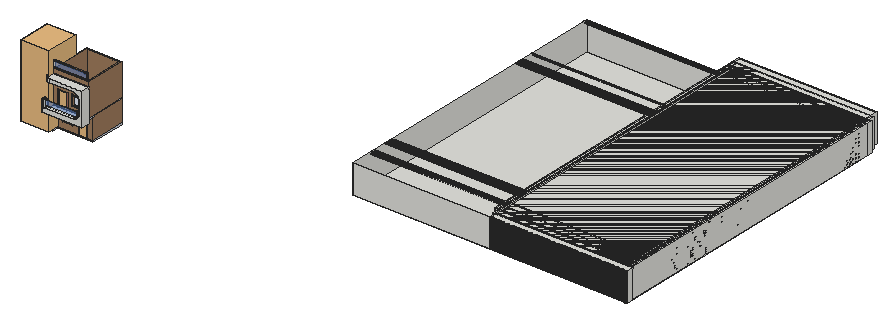
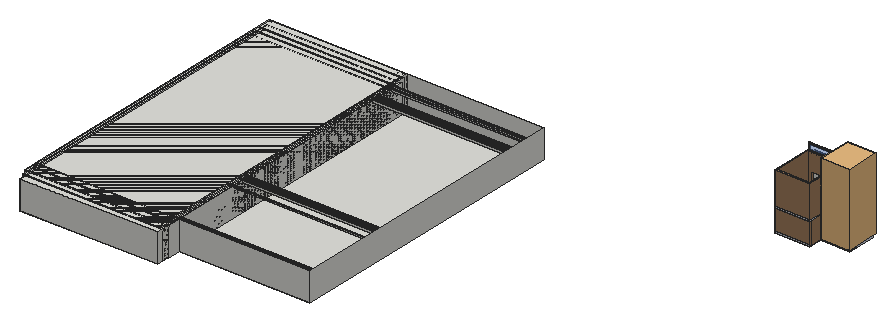
# SketchUp Ruby script. Lengths in inches.
U = 1.inch
M = Sketchup.active_model
def pt(a) = Geom::Point3d.new(a.map { |v| v * U })
def face(e, loops, mat)
  f = e.add_face(loops[0].map { |a| pt(a) })
  loops[1..].each { |l| e.add_face(l.map { |a| pt(a) }).erase! }
  f.material = f.back_material = mat if mat
  f
end
# faces: each face lists its corners as indices into pts; further lists are holes
def faces(e, pts, list, mat = nil) = list.each { |f| face(e, (f[0].is_a?(Array) ? f : [f]).map { |l| l.map { |i| pts[i] } }, mat) }
# xy, xz, yz: faces in a plane at the given z, y or x. An outline is a flat list of corners, or four numbers for a rectangle; further outlines are holes
def ring(l) = l.size == 4 ? [[l[0], l[1]], [l[2], l[1]], [l[2], l[3]], [l[0], l[3]]] : l.each_slice(2).to_a
def flat(e, list, mat, &to3) = list.each { |f| face(e, (f[0].is_a?(Array) ? f : [f]).map { |l| ring(l).map { |u, v| to3.(u, v) } }, mat) }
def xy(e, z, list, mat = nil) = flat(e, list, mat) { |x, y| [x, y, z] }
def xz(e, y, list, mat = nil) = flat(e, list, mat) { |x, z| [x, y, z] }
def yz(e, x, list, mat = nil) = flat(e, list, mat) { |y, z| [x, y, z] }
def lines(e, pts, list) = list.each { |a, b| e.add_line(pt(pts[a]), pt(pts[b])) }
# prism: a flat outline (further loops are holes) pulled along v
def prism(e, loops, v, mat = nil)
  f = face(e, loops, mat); d = Geom::Vector3d.new(v.map { |x| x * U })
  f.pushpull(f.normal.samedirection?(d) ? d.length : -d.length)
end
def box(e, o, s, mat = nil) = prism(e, [[o, [o[0] + s[0], o[1], o[2]], [o[0] + s[0], o[1] + s[1], o[2]], [o[0], o[1] + s[1], o[2]]]], [0, 0, s[2]], mat)
def at(x, y, z, deg = 0) = Geom::Transformation.translation(pt([x, y, z])) * Geom::Transformation.rotation(ORIGIN, Z_AXIS, deg.degrees)
def axes(o, x, y, z) = Geom::Transformation.new([*x, 0, *y, 0, *z, 0, *pt(o).to_a, 1])
def part(name) = M.definitions.add(name)
# library, detail: a bought-in or finely detailed component or shape, given as its bounding box
def library(name, o, s) = part(name).tap { |d| box(d.entities, o, s) }
def detail(e, o, s) = box(e.add_group.entities, o, s)
def put(e, d, t, mat = nil) = e.add_instance(d, t).tap { |i| i.material = mat if mat }
def group(e, t, mat = nil) = e.add_group.tap { |g| g.transformation = t; g.material = mat if mat }.entities
root = M.entities
M.materials.add("[Cladding Siding Tan]").color = [162, 126, 95]
M.materials.add("[Marble Carrara Floor Tile]").color = [204, 208, 219]
M.materials.add("[Stone Flagstone Ashlar]").color = [175, 116, 102]
M.materials.add("[Translucent Glass Blue]").color = [100, 149, 237]
M.materials["[Translucent Glass Blue]"].alpha = 0.5
c1 = part("Group478\#1")
prism(c1.entities,[[[385.16,-80.25,5.875],[385.16,-76.86,0],[385.16,-75.67,0],[385.16,-79.0625,5.875]]],[-770.3125,0,0])
c2 = part("Group479\#1")
prism(c2.entities,[[[385.16,-76.3125,5.875],[385.16,-72.92,0],[385.16,-71.73,0],[385.16,-75.125,5.875]]],[-770.3125,0,0])
c3 = part("Group480\#1")
prism(c3.entities,[[[385.16,-68.98,0],[385.16,-67.8,0],[385.16,-71.1875,5.875],[385.16,-72.375,5.875]]],[-770.3125,0,0])
c4 = part("Group481\#1")
prism(c4.entities,[[[-385.16,-63.86,0],[-385.16,-65.05,0],[-385.16,-68.4375,5.875],[-385.16,-67.25,5.875]]],[770.3125,0,0])
c5 = part("Group482\#1")
prism(c5.entities,[[[-385.16,-59.92,0],[-385.16,-61.11,0],[-385.16,-64.5,5.875],[-385.16,-63.3125,5.875]]],[770.3125,0,0])
c6 = part("Group483\#1")
prism(c6.entities,[[[385.16,-59.375,5.875],[385.16,-60.5625,5.875],[385.16,-57.17,0],[385.16,-55.98,0]]],[-770.3125,0,0])
c7 = part("Group484\#1")
prism(c7.entities,[[[385.16,-56.625,5.875],[385.16,-53.23,0],[385.16,-52.05,0],[385.16,-55.4375,5.875]]],[-770.3125,0,0])
c8 = part("Group485\#1")
prism(c8.entities,[[[385.16,-52.6875,5.875],[385.16,-49.3,0],[385.16,-48.11,0],[385.16,-51.5,5.875]]],[-770.3125,0,0])
c9 = part("Group486\#1")
prism(c9.entities,[[[-385.16,-48.75,5.875],[-385.16,-47.5625,5.875],[-385.16,-44.17,0],[-385.16,-45.36,0]]],[770.3125,0,0])
c10 = part("Group487\#1")
prism(c10.entities,[[[-385.16,-41.42,0],[-385.16,-44.8125,5.875],[-385.16,-43.625,5.875],[-385.16,-40.23,0]]],[770.3125,0,0])
c11 = part("Group488\#1")
prism(c11.entities,[[[385.16,-37.48,0],[385.16,-36.3,0],[385.16,-39.6875,5.875],[385.16,-40.875,5.875]]],[-770.3125,0,0])
c12 = part("Group489\#1")
prism(c12.entities,[[[385.16,-33.55,0],[385.16,-32.36,0],[385.16,-35.75,5.875],[385.16,-36.9375,5.875]]],[-770.3125,0,0])
c13 = part("Group490\#1")
prism(c13.entities,[[[385.16,-33,5.875],[385.16,-29.61,0],[385.16,-28.42,0],[385.16,-31.8125,5.875]]],[-770.3125,0,0])
c14 = part("Group491\#1")
prism(c14.entities,[[[385.16,-24.48,0],[385.16,-27.875,5.875],[385.16,-29.0625,5.875],[385.16,-25.67,0]]],[-770.3125,0,0])
c15 = part("Group492\#1")
prism(c15.entities,[[[-385.16,-25.125,5.875],[-385.16,-23.9375,5.875],[-385.16,-20.55,0],[-385.16,-21.73,0]]],[770.3125,0,0])
c16 = part("Group493\#1")
prism(c16.entities,[[[385.16,-21.1875,5.875],[385.16,-17.8,0],[385.16,-16.61,0],[385.16,-20,5.875]]],[-770.3125,0,0])
c17 = part("Group494\#1")
prism(c17.entities,[[[385.16,-13.86,0],[385.16,-12.67,0],[385.16,-16.0625,5.875],[385.16,-17.25,5.875]]],[-770.3125,0,0])
c18 = part("Group495\#1")
prism(c18.entities,[[[-385.16,-13.3125,5.875],[-385.16,-12.125,5.875],[-385.16,-8.73,0],[-385.16,-9.92,0]]],[770.3125,0,0])
c19 = part("Group496\#1")
prism(c19.entities,[[[385.16,-9.375,5.875],[385.16,-5.98,0],[385.16,-4.8,0],[385.16,-8.1875,5.875]]],[-770.3125,0,0])
c20 = part("Group497\#1")
prism(c20.entities,[[[385.16,-0.86,0],[385.16,-4.25,5.875],[385.16,-5.4375,5.875],[385.16,-2.05,0]]],[-770.3125,0,0])
c21 = part("Group498\#1")
prism(c21.entities,[[[-385.16,-1.5,5.875],[-385.16,-0.3125,5.875],[-385.16,3.08,0],[-385.16,1.89,0]]],[770.3125,0,0])
c22 = part("Group499\#1")
prism(c22.entities,[[[385.16,5.83,0],[385.16,7.02,0],[385.16,3.625,5.875],[385.16,2.4375,5.875]]],[-770.3125,0,0])
c23 = part("Group500\#1")
prism(c23.entities,[[[-385.16,9.77,0],[-385.16,6.375,5.875],[-385.16,7.5625,5.875],[-385.16,10.95,0]]],[770.3125,0,0])
c24 = part("Group501\#1")
prism(c24.entities,[[[-385.16,14.89,0],[-385.16,13.7,0],[-385.16,10.3125,5.875],[-385.16,11.5,5.875]]],[770.3125,0,0])
c25 = part("Group502\#1")
prism(c25.entities,[[[-385.16,15.4375,5.875],[-385.16,18.83,0],[-385.16,17.64,0],[-385.16,14.25,5.875]]],[770.3125,0,0])
c26 = part("Group503\#1")
prism(c26.entities,[[[385.16,19.375,5.875],[385.16,18.1875,5.875],[385.16,21.58,0],[385.16,22.77,0]]],[-770.3125,0,0])
c27 = part("Group504\#1")
prism(c27.entities,[[[-385.16,26.7,0],[-385.16,25.52,0],[-385.16,22.125,5.875],[-385.16,23.3125,5.875]]],[770.3125,0,0])
c28 = part("Group505\#1")
prism(c28.entities,[[[385.16,29.45,0],[385.16,30.64,0],[385.16,27.25,5.875],[385.16,26.0625,5.875]]],[-770.3125,0,0])
c29 = part("Group506\#1")
prism(c29.entities,[[[-385.16,33.39,0],[-385.16,30,5.875],[-385.16,31.1875,5.875],[-385.16,34.58,0]]],[770.3125,0,0])
c30 = part("Group507\#1")
prism(c30.entities,[[[385.16,33.9375,5.875],[385.16,37.33,0],[385.16,38.52,0],[385.16,35.125,5.875]]],[-770.3125,0,0])
c31 = part("Group508\#1")
prism(c31.entities,[[[-385.16,42.45,0],[-385.16,41.27,0],[-385.16,37.875,5.875],[-385.16,39.0625,5.875]]],[770.3125,0,0])
c32 = part("Group509\#1")
prism(c32.entities,[[[385.16,46.39,0],[385.16,43,5.875],[385.16,41.8125,5.875],[385.16,45.2,0]]],[-770.3125,0,0])
c33 = part("Group510\#1")
prism(c33.entities,[[[-385.16,49.14,0],[-385.16,45.75,5.875],[-385.16,46.9375,5.875],[-385.16,50.33,0]]],[770.3125,0,0])
c34 = part("Group511\#1")
prism(c34.entities,[[[385.16,50.875,5.875],[385.16,49.6875,5.875],[385.16,53.08,0],[385.16,54.27,0]]],[-770.3125,0,0])
c35 = part("Group512\#1")
prism(c35.entities,[[[385.16,54.8125,5.875],[385.16,53.625,5.875],[385.16,57.02,0],[385.16,58.2,0]]],[-770.3125,0,0])
c36 = part("Group513\#1")
prism(c36.entities,[[[385.16,62.14,0],[385.16,58.75,5.875],[385.16,57.5625,5.875],[385.16,60.95,0]]],[-770.3125,0,0])
c37 = part("Group514\#1")
prism(c37.entities,[[[-385.16,62.6875,5.875],[-385.16,66.08,0],[-385.16,64.89,0],[-385.16,61.5,5.875]]],[770.3125,0,0])
c38 = part("Group515\#1")
prism(c38.entities,[[[-385.16,70.02,0],[-385.16,68.83,0],[-385.16,65.4375,5.875],[-385.16,66.625,5.875]]],[770.3125,0,0])
c39 = part("Group516\#1")
prism(c39.entities,[[[385.16,72.77,0],[385.16,73.95,0],[385.16,70.5625,5.875],[385.16,69.375,5.875]]],[-770.3125,0,0])
c40 = part("Group517\#1")
prism(c40.entities,[[[385.16,76.7,0],[385.16,77.89,0],[385.16,74.5,5.875],[385.16,73.3125,5.875]]],[-770.3125,0,0])
c41 = part("Group518\#1")
xy(c41.entities,5.875,[[-385.16,77.25,385.16,78.4375]])
p = [[385.16,77.25,5.875],[-385.16,77.25,5.875],[-385.16,80.25,0.68],[385.16,80.25,0.68],[-385.16,78.4375,5.875],[385.16,78.4375,5.875],
  [385.16,80.25,2.74],[-385.16,80.25,2.74]]
faces(c41.entities,p,[[0,1,2,3],[4,5,6,7]])
c42 = part("Group476\#2")
put(c42.entities,c1,at(0,0,0))
put(c42.entities,c2,at(0,0,0))
put(c42.entities,c3,at(0,0,0))
put(c42.entities,c4,at(0,0,0))
put(c42.entities,c5,at(0,0,0))
put(c42.entities,c6,at(0,0,0))
put(c42.entities,c7,at(0,0,0))
put(c42.entities,c8,at(0,0,0))
put(c42.entities,c9,at(0,0,0))
put(c42.entities,c10,at(0,0,0))
put(c42.entities,c11,at(0,0,0))
put(c42.entities,c12,at(0,0,0))
put(c42.entities,c13,at(0,0,0))
put(c42.entities,c14,at(0,0,0))
put(c42.entities,c15,at(0,0,0))
put(c42.entities,c16,at(0,0,0))
put(c42.entities,c17,at(0,0,0))
put(c42.entities,c18,at(0,0,0))
put(c42.entities,c19,at(0,0,0))
put(c42.entities,c20,at(0,0,0))
put(c42.entities,c21,at(0,0,0))
put(c42.entities,c22,at(0,0,0))
put(c42.entities,c23,at(0,0,0))
put(c42.entities,c24,at(0,0,0))
put(c42.entities,c25,at(0,0,0))
put(c42.entities,c26,at(0,0,0))
put(c42.entities,c27,at(0,0,0))
put(c42.entities,c28,at(0,0,0))
put(c42.entities,c29,at(0,0,0))
put(c42.entities,c30,at(0,0,0))
put(c42.entities,c31,at(0,0,0))
put(c42.entities,c32,at(0,0,0))
put(c42.entities,c33,at(0,0,0))
put(c42.entities,c34,at(0,0,0))
put(c42.entities,c35,at(0,0,0))
put(c42.entities,c36,at(0,0,0))
put(c42.entities,c37,at(0,0,0))
put(c42.entities,c38,at(0,0,0))
put(c42.entities,c39,at(0,0,0))
put(c42.entities,c40,at(0,0,0))
put(c42.entities,c41,at(0,0,0))
c43 = library("Group1\#1",[84,59.0625,0],[162,188.875,405.6875])
c44 = library("Group\#3",[0,0,0],[54.125,9.07,48])
c45 = library("Group\#4",[0,0,0],[48.61,10.47,82])
c46 = part("Group14\#2")
xy(c46.entities,120,[[246,116.375,246,310.5625,255,310.5625,255,125.375,438,125.375,438,310.5625,246,310.5625,246,319.5625,447,319.5625,447,116.375]],"[Cladding Siding Tan]")
xy(c46.entities,123,[[364.6,116.375,413.22,125.375]],"[Cladding Siding Tan]")
xy(c46.entities,156,[[275.96,116.375,330.08,125.375]],"[Cladding Siding Tan]")
xy(c46.entities,204,[[275.96,116.375,330.08,125.375]],"[Cladding Siding Tan]")
xy(c46.entities,205,[[364.6,116.375,413.22,125.375]],"[Cladding Siding Tan]")
xy(c46.entities,240,[[246,116.375,447,116.375,447,319.5625,246,319.5625,246,310.5625,438,310.5625,438,125.375,255,125.375,255,310.5625,246,310.5625]],"[Cladding Siding Tan]")
xz(c46.entities,116.375,[[[246,120,447,240],[364.6,123,413.22,205],[275.96,156,330.08,204]]],"[Cladding Siding Tan]")
xz(c46.entities,125.375,[[[255,120,438,240],[364.6,123,413.22,205],[275.96,156,330.08,204]]],"[Cladding Siding Tan]")
xz(c46.entities,310.5625,[[246,120,255,240],[255,120,438,240]],"[Cladding Siding Tan]")
xz(c46.entities,319.5625,[[246,120,447,240]],"[Cladding Siding Tan]")
yz(c46.entities,246,[[116.375,120,310.5625,240],[310.5625,120,319.5625,240]],"[Cladding Siding Tan]")
yz(c46.entities,255,[[125.375,120,310.5625,240]],"[Cladding Siding Tan]")
yz(c46.entities,275.96,[[116.375,156,125.375,204]],"[Cladding Siding Tan]")
yz(c46.entities,330.08,[[116.375,156,125.375,204]],"[Cladding Siding Tan]")
yz(c46.entities,364.6,[[116.375,123,125.375,205]],"[Cladding Siding Tan]")
yz(c46.entities,413.22,[[116.375,123,125.375,205]],"[Cladding Siding Tan]")
yz(c46.entities,438,[[125.375,120,310.5625,240]],"[Cladding Siding Tan]")
yz(c46.entities,447,[[116.375,120,319.5625,240]],"[Cladding Siding Tan]")
put(c46.entities,c44,at(275.96,116.375,156))
put(c46.entities,c45,at(364.6,114.9,123))
c47 = library("Group\#5",[0,0,0],[45.42,10.47,82])
c48 = part("Group24\#1")
box(c48.entities,[247.82,89.26,308.1875],[2.36,2.36,41.54])
c49 = part("Group25\#1")
box(c49.entities,[434.07,89.26,308.1875],[2.36,2.36,41.54])
c50 = part("Group27\#1")
box(c50.entities,[247.82,89.06,349.73],[188.61,2.76,1.77])
c51 = part("Group28\#1")
box(c51.entities,[249,89.45,344.61],[186.25,1.97,0.98])
c52 = part("Group29\#1")
box(c52.entities,[249,89.45,313.11],[186.25,1.97,0.98])
c53 = part("Group30\#1")
xz(c53.entities,90.4375,[[249,314.09,435.25,344.61]],"[Translucent Glass Blue]")
c54 = part("Group30\#2")
prism(c54.entities,[[[236.9,48.19,127.08],[239.26,48.17,127.08],[239.24,45.8,127.08],[236.875,45.83,127.08]]],[0,0,41.54])
c55 = part("Group31\#1")
prism(c55.entities,[[[413.05,46.48,130.48],[415.42,46.45,130.48],[415.39,44.09,130.48],[413.03,44.11,130.48]]],[0,0,41.54])
c56 = part("Group34\#1")
prism(c56.entities,[[[414.21,44.3,167.89],[238.06,46.01,164.49],[238.06,46.01,163.5],[414.21,44.3,166.91]]],[0.02,1.97,0])
c57 = part("Group35\#1")
prism(c57.entities,[[[414.21,44.3,136.39],[238.06,46.01,132.99],[238.06,46.01,132],[414.21,44.3,135.4]]],[0.02,1.97,0])
c58 = part("Group36\#1")
p = [[238.07,47,163.5],[238.07,47,132.99],[414.22,45.28,136.39],[414.22,45.28,166.91]]
faces(c58.entities,p,[[0,1,2,3]],"[Translucent Glass Blue]")
c59 = part("Group12\#1")
xy(c59.entities,99.72,[[219.83,190.5,447,238.9375]],"[Cladding Siding Tan]")
xy(c59.entities,126,[[274.58,235.9375,274.58,238.9375,246,238.9375,246,247.9375,438,247.9375,438,463.9375,255,463.9375,255,247.9375,246,247.9375,246,472.9375,447,472.9375,447,238.9375,328,238.9375,328,235.9375,324,235.9375,324,238.9375,278.58,238.9375,278.58,235.9375]],"[Cladding Siding Tan]")
xy(c59.entities,127.08,[[234.69,190.5,397.22,238.9375]])
xy(c59.entities,129,[[278.58,238.9375,324,247.9375]],"[Cladding Siding Tan]")
xy(c59.entities,157.39,[[352.34,235.9375,424.28,238.9375]],"[Cladding Siding Tan]")
xy(c59.entities,162,[[357.34,235.9375,419.67,247.9375]],"[Cladding Siding Tan]")
xy(c59.entities,168.02,[[219.83,190.5,234.69,238.9375]])
xy(c59.entities,210,[[357.34,235.9375,419.67,247.9375]],"[Cladding Siding Tan]")
xy(c59.entities,211,[[278.58,235.9375,324,247.9375]],"[Cladding Siding Tan]")
xy(c59.entities,215,[[274.58,235.9375,328,238.9375],[352.34,235.9375,424.28,238.9375]],"[Stone Flagstone Ashlar]")
xy(c59.entities,264.4375,[[268.89,190.5,257.17,191.56,247.59,194.76,240.13,200.08,234.81,207.54,231.61,217.125,230.55,228.84,230.55,238.9375,389.06,238.9375,389.06,190.5]])
xy(c59.entities,283.86,[[268.89,190.5,447,190.5,447,238.9375,230.55,238.9375,230.55,228.84,231.61,217.125,234.81,207.54,240.13,200.08,247.59,194.76,257.17,191.56]])
xy(c59.entities,308.1875,[[[246,238.9375,447,472.9375],[255,247.9375,438,463.9375]]],"[Cladding Siding Tan]")
xz(c59.entities,190.5,[[219.83,99.72,447,99.72,447,283.86,268.89,283.86,268.89,264.4375,389.06,264.4375,400.9,263.36,410.6,260.13,418.13,254.75,423.52,247.21,426.75,237.52,427.83,225.67,427.83,157.6875,426.98,148.34,424.43,140.68,420.18,134.73,414.22,130.48,406.57,127.93,397.22,127.08,234.69,127.08,234.69,168.02,219.83,168.02]])
xz(c59.entities,235.9375,[[274.58,126,278.58,126,278.58,211,324,211,324,126,328,126,328,215,274.58,215],[[352.34,157.39,424.28,215],[357.34,162,419.67,210]]],"[Stone Flagstone Ashlar]")
xz(c59.entities,238.9375,[[219.83,99.72,219.83,168.02,234.69,168.02,234.69,127.08,246,127.08,246,126,274.58,126,274.58,127.08,278.58,127.08,278.58,126,324,126,324,127.08,328,127.08,328,126,427.83,126,427.83,99.72],[427.83,99.72,447,126],[246,126,274.58,127.08],[427.83,126,447,126,447,283.86,246,283.86,246,264.4375,427.83,264.4375],[278.58,126,324,127.08],
  [328,126,328,127.08,397.22,127.08,406.57,127.93,414.22,130.48,420.18,134.73,424.43,140.68,426.98,148.34,427.83,157.6875,427.83,126],[[246,127.08,274.58,127.08,274.58,215,328,215,328,127.08,397.22,127.08,406.57,127.93,414.22,130.48,420.18,134.73,424.43,140.68,426.98,148.34,427.83,157.6875,427.83,225.67,426.75,237.52,423.52,247.21,418.13,254.75,410.6,260.13,400.9,263.36,389.06,264.4375,246,264.4375],[352.34,157.39,424.28,215]],[278.58,127.08,324,129],[427.83,225.67,426.75,237.52,423.52,247.21,418.13,254.75,410.6,260.13,400.9,263.36,389.06,264.4375,427.83,264.4375],[230.55,264.4375,246,283.86],
  [246,283.86,447,308.1875]],"[Cladding Siding Tan]")
xz(c59.entities,247.9375,[[246,126,255,246],[[255,126,438,308.1875],[278.58,129,324,211],[357.34,162,419.67,210]]],"[Cladding Siding Tan]")
xz(c59.entities,463.9375,[[255,126,438,308.1875]],"[Cladding Siding Tan]")
xz(c59.entities,472.9375,[[246,126,447,308.1875]],"[Cladding Siding Tan]")
yz(c59.entities,219.83,[[190.5,99.72,238.9375,168.02]])
yz(c59.entities,230.55,[[228.84,264.4375,238.9375,283.86]])
yz(c59.entities,234.69,[[190.5,127.08,238.9375,168.02]])
yz(c59.entities,246,[[238.9375,126,247.9375,308.1875],[247.9375,126,472.9375,308.1875]],"[Cladding Siding Tan]")
yz(c59.entities,255,[[247.9375,126,463.9375,308.1875]],"[Cladding Siding Tan]")
yz(c59.entities,274.58,[[235.9375,126,238.9375,215]],"[Stone Flagstone Ashlar]")
yz(c59.entities,278.58,[[235.9375,126,238.9375,129],[235.9375,129,247.9375,211]],"[Cladding Siding Tan]")
yz(c59.entities,324,[[235.9375,126,238.9375,129],[235.9375,129,247.9375,211]],"[Cladding Siding Tan]")
yz(c59.entities,328,[[235.9375,126,238.9375,215]],"[Stone Flagstone Ashlar]")
yz(c59.entities,352.34,[[235.9375,157.39,238.9375,215]],"[Stone Flagstone Ashlar]")
yz(c59.entities,357.34,[[235.9375,162,247.9375,210]],"[Cladding Siding Tan]")
yz(c59.entities,419.67,[[235.9375,162,247.9375,210]],"[Cladding Siding Tan]")
yz(c59.entities,424.28,[[235.9375,157.39,238.9375,215]],"[Cladding Siding Tan]")
yz(c59.entities,427.83,[[190.5,157.6875,238.9375,225.67]])
yz(c59.entities,438,[[247.9375,126,463.9375,308.1875]],"[Cladding Siding Tan]")
yz(c59.entities,447,[[190.5,99.72,238.9375,283.86]])
yz(c59.entities,447,[[238.9375,126,472.9375,308.1875]],"[Cladding Siding Tan]")
p = [[397.22,238.9375,127.08],[397.22,190.5,127.08],[406.57,190.5,127.93],[406.57,238.9375,127.93],[414.22,190.5,130.48],[414.22,198.28,130.48],
  [414.22,238.9375,130.48],[420.18,190.5,134.73],[420.18,238.9375,134.73],[424.43,190.5,140.68],[424.43,238.9375,140.68],[426.98,190.5,148.34],
  [426.98,238.9375,148.34],[427.83,190.5,157.6875],[427.83,238.9375,157.6875],[427.83,238.9375,225.67],[427.83,190.5,225.67],[426.75,190.5,237.52],
  [426.75,238.9375,237.52],[423.52,190.5,247.21],[423.52,238.9375,247.21],[418.13,190.5,254.75],[418.13,238.9375,254.75],[410.6,190.5,260.13],
  [410.6,238.9375,260.13],[400.9,190.5,263.36],[400.9,238.9375,263.36],[389.06,190.5,264.4375],[389.06,238.9375,264.4375],[257.17,191.56,283.86],
  [257.17,191.56,264.4375],[268.89,190.5,264.4375],[268.89,190.5,283.86],[247.59,194.76,283.86],[247.59,194.76,264.4375],[240.13,200.08,283.86],
  [240.13,200.08,264.4375],[234.81,207.54,283.86],[234.81,207.54,264.4375],[231.61,217.125,283.86],[231.61,217.125,264.4375],[230.55,228.84,283.86],
  [230.55,228.84,264.4375]]
faces(c59.entities,p,[[0,1,2,3],[3,2,4,5,6],[5,4,7,8,6],[8,7,9,10],[10,9,11,12],[12,11,13,14],[15,16,17,18],[18,17,19,20],
  [20,19,21,22],[22,21,23,24],[24,23,25,26],[26,25,27,28],[29,30,31,32],[33,34,30,29],[35,36,34,33],[37,38,36,35],
  [39,40,38,37],[41,42,40,39]])
put(c59.entities,c47,at(278.58,237.47,129))
put(c59.entities,c48,axes([-192.56,153,0],[1.76967,0,0],[0,1,0],[0,0,1]))
put(c59.entities,c49,axes([-288.4375,197.63,0],[1.6645,0,0],[0,0.5,0],[0,0,1]))
put(c59.entities,c50,axes([-6.27,153,0],[1.01796,0,0],[0,1,0],[0,0,1]))
put(c59.entities,c51,at(0,153,0))
put(c59.entities,c52,at(0,153,0))
put(c59.entities,c53,at(0,153,0))
put(c59.entities,c54,axes([-219.25,153,1.85],[1.91634,0,0],[0,1,0],[0,0,0.98548]))
put(c59.entities,c55,axes([-128.04,153,1.3],[1.31,0,0],[0,1,0],[0,0,0.99]))
put(c59.entities,c56,at(0,153,0))
put(c59.entities,c57,at(0,153,0))
put(c59.entities,c58,at(0,153,0))
c60 = part("Group471\#1")
p = [[385.16,799.33,0],[-385.16,799.33,0],[-385.16,795.9375,5.875],[385.16,795.9375,5.875]]
faces(c60.entities,p,[[0,1,2,3]])
c61 = part("Group473\#1")
p = [[-385.16,803.8125,5.875],[385.16,803.8125,5.875],[385.16,807.2,0],[-385.16,807.2,0]]
faces(c61.entities,p,[[0,1,2,3]])
c62 = part("Group475\#1")
p = [[385.16,815.08,0],[-385.16,815.08,0],[-385.16,811.6875,5.875],[385.16,811.6875,5.875]]
faces(c62.entities,p,[[0,1,2,3]])
c63 = part("Group351\#1")
p = [[-385.16,323.4375,5.875],[385.16,323.4375,5.875],[385.16,326.83,0],[-385.16,326.83,0]]
faces(c63.entities,p,[[0,1,2,3]])
c64 = part("Group352\#1")
p = [[-385.16,327.375,5.875],[385.16,327.375,5.875],[385.16,330.77,0],[-385.16,330.77,0]]
faces(c64.entities,p,[[0,1,2,3]])
c65 = part("Group353\#1")
p = [[385.16,334.7,0],[-385.16,334.7,0],[-385.16,331.3125,5.875],[385.16,331.3125,5.875]]
faces(c65.entities,p,[[0,1,2,3]])
c66 = part("Group354\#1")
p = [[-385.16,335.25,5.875],[385.16,335.25,5.875],[385.16,338.64,0],[-385.16,338.64,0]]
faces(c66.entities,p,[[0,1,2,3]])
c67 = part("Group355\#1")
p = [[385.16,342.58,0],[-385.16,342.58,0],[-385.16,339.1875,5.875],[385.16,339.1875,5.875]]
faces(c67.entities,p,[[0,1,2,3]])
c68 = part("Group356\#1")
p = [[385.16,346.52,0],[-385.16,346.52,0],[-385.16,343.125,5.875],[385.16,343.125,5.875]]
faces(c68.entities,p,[[0,1,2,3]])
c69 = part("Group357\#1")
p = [[-385.16,347.0625,5.875],[385.16,347.0625,5.875],[385.16,350.45,0],[-385.16,350.45,0]]
faces(c69.entities,p,[[0,1,2,3]])
c70 = part("Group358\#1")
p = [[385.16,354.39,0],[-385.16,354.39,0],[-385.16,351,5.875],[385.16,351,5.875]]
faces(c70.entities,p,[[0,1,2,3]])
c71 = part("Group359\#1")
p = [[385.16,358.33,0],[-385.16,358.33,0],[-385.16,354.9375,5.875],[385.16,354.9375,5.875]]
faces(c71.entities,p,[[0,1,2,3]])
c72 = part("Group360\#1")
p = [[-385.16,358.875,5.875],[385.16,358.875,5.875],[385.16,362.27,0],[-385.16,362.27,0]]
faces(c72.entities,p,[[0,1,2,3]])
c73 = part("Group361\#1")
p = [[-385.16,362.8125,5.875],[385.16,362.8125,5.875],[385.16,366.2,0],[-385.16,366.2,0]]
faces(c73.entities,p,[[0,1,2,3]])
c74 = part("Group362\#1")
p = [[-385.16,366.75,5.875],[385.16,366.75,5.875],[385.16,370.14,0],[-385.16,370.14,0]]
faces(c74.entities,p,[[0,1,2,3]])
c75 = part("Group363\#1")
p = [[-385.16,370.6875,5.875],[385.16,370.6875,5.875],[385.16,374.08,0],[-385.16,374.08,0]]
faces(c75.entities,p,[[0,1,2,3]])
c76 = part("Group364\#1")
p = [[385.16,378.02,0],[-385.16,378.02,0],[-385.16,374.625,5.875],[385.16,374.625,5.875]]
faces(c76.entities,p,[[0,1,2,3]])
c77 = part("Group379\#1")
p = [[385.16,437.08,0],[-385.16,437.08,0],[-385.16,433.6875,5.875],[385.16,433.6875,5.875]]
faces(c77.entities,p,[[0,1,2,3]])
c78 = part("Group380\#1")
p = [[-385.16,437.625,5.875],[385.16,437.625,5.875],[385.16,441.02,0],[-385.16,441.02,0]]
faces(c78.entities,p,[[0,1,2,3]])
c79 = part("Group91\#1")
p = [[385.16,-696.92,0],[-385.16,-696.92,0],[-385.16,-700.3125,5.875],[385.16,-700.3125,5.875]]
faces(c79.entities,p,[[0,1,2,3]])
c80 = part("Group93\#1")
p = [[385.16,-689.05,0],[-385.16,-689.05,0],[-385.16,-692.4375,5.875],[385.16,-692.4375,5.875]]
faces(c80.entities,p,[[0,1,2,3]])
c81 = part("Group95\#1")
p = [[-385.16,-684.5625,5.875],[385.16,-684.5625,5.875],[385.16,-681.17,0],[-385.16,-681.17,0]]
faces(c81.entities,p,[[0,1,2,3]])
c82 = part("Group97\#1")
p = [[385.16,-673.3,0],[-385.16,-673.3,0],[-385.16,-676.6875,5.875],[385.16,-676.6875,5.875]]
faces(c82.entities,p,[[0,1,2,3]])
c83 = part("Group99\#1")
p = [[385.16,-665.42,0],[-385.16,-665.42,0],[-385.16,-668.8125,5.875],[385.16,-668.8125,5.875]]
faces(c83.entities,p,[[0,1,2,3]])
c84 = part("Group118\#1")
p = [[-385.16,-594,5.875],[385.16,-594,5.875],[385.16,-590.61,0],[-385.16,-590.61,0]]
faces(c84.entities,p,[[0,1,2,3]])
c85 = part("Group119\#1")
p = [[385.16,-586.67,0],[-385.16,-586.67,0],[-385.16,-590.0625,5.875],[385.16,-590.0625,5.875]]
faces(c85.entities,p,[[0,1,2,3]])
c86 = part("Group120\#1")
p = [[-385.16,-586.125,5.875],[385.16,-586.125,5.875],[385.16,-582.73,0],[-385.16,-582.73,0]]
faces(c86.entities,p,[[0,1,2,3]])
c87 = part("Group121\#1")
p = [[385.16,-578.8,0],[-385.16,-578.8,0],[-385.16,-582.1875,5.875],[385.16,-582.1875,5.875]]
faces(c87.entities,p,[[0,1,2,3]])
c88 = part("Group122\#1")
p = [[-385.16,-578.25,5.875],[385.16,-578.25,5.875],[385.16,-574.86,0],[-385.16,-574.86,0]]
faces(c88.entities,p,[[0,1,2,3]])
c89 = part("Group123\#1")
p = [[385.16,-570.92,0],[-385.16,-570.92,0],[-385.16,-574.3125,5.875],[385.16,-574.3125,5.875]]
faces(c89.entities,p,[[0,1,2,3]])
c90 = part("Group124\#1")
p = [[385.16,-566.98,0],[-385.16,-566.98,0],[-385.16,-570.375,5.875],[385.16,-570.375,5.875]]
faces(c90.entities,p,[[0,1,2,3]])
c91 = part("Group125\#1")
p = [[-385.16,-566.4375,5.875],[385.16,-566.4375,5.875],[385.16,-563.05,0],[-385.16,-563.05,0]]
faces(c91.entities,p,[[0,1,2,3]])
c92 = part("Group126\#1")
p = [[-385.16,-562.5,5.875],[385.16,-562.5,5.875],[385.16,-559.11,0],[-385.16,-559.11,0]]
faces(c92.entities,p,[[0,1,2,3]])
c93 = part("Group127\#1")
p = [[-385.16,-558.5625,5.875],[385.16,-558.5625,5.875],[385.16,-555.17,0],[-385.16,-555.17,0]]
faces(c93.entities,p,[[0,1,2,3]])
c94 = part("Group128\#1")
p = [[385.16,-551.23,0],[-385.16,-551.23,0],[-385.16,-554.625,5.875],[385.16,-554.625,5.875]]
faces(c94.entities,p,[[0,1,2,3]])
c95 = part("Group129\#1")
p = [[385.16,-547.3,0],[-385.16,-547.3,0],[-385.16,-550.6875,5.875],[385.16,-550.6875,5.875]]
faces(c95.entities,p,[[0,1,2,3]])
c96 = part("Group130\#1")
p = [[-385.16,-546.75,5.875],[385.16,-546.75,5.875],[385.16,-543.36,0],[-385.16,-543.36,0]]
faces(c96.entities,p,[[0,1,2,3]])
c97 = part("Group131\#1")
p = [[-385.16,-542.8125,5.875],[385.16,-542.8125,5.875],[385.16,-539.42,0],[-385.16,-539.42,0]]
faces(c97.entities,p,[[0,1,2,3]])
c98 = part("Group132\#1")
p = [[-385.16,-538.875,5.875],[385.16,-538.875,5.875],[385.16,-535.48,0],[-385.16,-535.48,0]]
faces(c98.entities,p,[[0,1,2,3]])
xy(root,-6,[[0,48.4375,162,210.4375],[162,79.25,363,282.4375]])
xy(root,0,[[0,48.4375,162,210.4375],[162,79.25,363,282.4375],[1552.78,414.02,2323.09,2050.9]])
xz(root,48.4375,[[0,-6,162,0]],"[Marble Carrara Floor Tile]")
xz(root,79.25,[[162,-6,363,0]],"[Marble Carrara Floor Tile]")
xz(root,210.4375,[[0,-6,162,0]],"[Marble Carrara Floor Tile]")
xz(root,282.4375,[[162,-6,363,0]],"[Marble Carrara Floor Tile]")
xz(root,414.02,[[1552.78,0,2323.09,160.5]])
xz(root,2050.9,[[1552.78,0,2323.09,160.5]])
yz(root,0,[[48.4375,-6,210.4375,0]],"[Marble Carrara Floor Tile]")
yz(root,162,[[79.25,-6,210.4375,0]])
yz(root,162,[[48.4375,-6,79.25,0],[210.4375,-6,282.4375,0]],"[Marble Carrara Floor Tile]")
yz(root,363,[[79.25,-6,282.4375,0]],"[Marble Carrara Floor Tile]")
yz(root,1552.78,[[414.02,0,2050.9,160.5]])
yz(root,2323.09,[[414.02,0,2050.9,160.5]])
g1 = group(root,at(2323.09,414.02,0))
xy(g1,0,[[0,0,770.3125,1636.875]])
xy(g1,160.5,[[0,0,770.3125,1636.875]])
xz(g1,1636.875,[[0,0,770.3125,160.5]])
yz(g1,0,[[0,0,1636.875,160.5]])
yz(g1,770.3125,[[0,0,1636.875,160.5]])
put(g1,c42,axes([385.16,2.9375,80.25],[1,0,0],[0,0,1],[0,-1,0]))
put(root,c43,at(-84,-37.5,0))
g2 = group(root,at(2323.09,453.4,0))
box(g2,[0,0,0],[770.3125,1636.875,160.5])
g3 = group(root,at(2323.09,492.77,0))
box(g3,[0,0,0],[770.3125,1636.875,160.5])
g4 = group(root,at(2306.32,449.65,0))
box(g4,[0,0,0],[770.3125,1636.875,160.5])
g5 = group(root,at(2306.32,489.03,0))
box(g5,[0,0,0],[770.3125,1636.875,160.5])
g6 = group(root,at(2306.32,528.4,0))
box(g6,[0,0,0],[770.3125,1636.875,160.5])
g7 = group(root,at(2289.56,485.28,0))
box(g7,[0,0,0],[770.3125,1636.875,160.5])
g8 = group(root,at(2289.56,524.65,0))
box(g8,[0,0,0],[770.3125,1636.875,160.5])
g9 = group(root,at(2289.56,564.03,0))
box(g9,[0,0,0],[770.3125,1636.875,160.5])
put(root,c46,at(-84,-37.125,-120))
put(root,c59,at(-84,-190.5,0))
g10 = group(root,at(162,48.4375,126),"[Marble Carrara Floor Tile]")
box(g10,[0,0,-6],[201,234,6])
put(root,c60,at(1937.93,1232.46,154.625))
put(root,c61,at(1937.93,1232.46,154.625))
put(root,c62,at(1937.93,1232.46,154.625))
put(root,c63,at(1937.93,1232.46,154.625))
put(root,c64,at(1937.93,1232.46,154.625))
put(root,c65,at(1937.93,1232.46,154.625))
put(root,c66,at(1937.93,1232.46,154.625))
put(root,c67,at(1937.93,1232.46,154.625))
put(root,c68,at(1937.93,1232.46,154.625))
put(root,c69,at(1937.93,1232.46,154.625))
put(root,c70,at(1937.93,1232.46,154.625))
put(root,c71,at(1937.93,1232.46,154.625))
put(root,c72,at(1937.93,1232.46,154.625))
put(root,c73,at(1937.93,1232.46,154.625))
put(root,c74,at(1937.93,1232.46,154.625))
put(root,c75,at(1937.93,1232.46,154.625))
put(root,c76,at(1937.93,1232.46,154.625))
put(root,c77,at(1937.93,1232.46,154.625))
put(root,c78,at(1937.93,1232.46,154.625))
put(root,c79,at(1937.93,1232.46,154.625))
put(root,c80,at(1937.93,1232.46,154.625))
put(root,c81,at(1937.93,1232.46,154.625))
put(root,c82,at(1937.93,1232.46,154.625))
put(root,c83,at(1937.93,1232.46,154.625))
put(root,c84,at(1937.93,1232.46,154.625))
put(root,c85,at(1937.93,1232.46,154.625))
put(root,c86,at(1937.93,1232.46,154.625))
put(root,c87,at(1937.93,1232.46,154.625))
put(root,c88,at(1937.93,1232.46,154.625))
put(root,c89,at(1937.93,1232.46,154.625))
put(root,c90,at(1937.93,1232.46,154.625))
put(root,c91,at(1937.93,1232.46,154.625))
put(root,c92,at(1937.93,1232.46,154.625))
put(root,c93,at(1937.93,1232.46,154.625))
put(root,c94,at(1937.93,1232.46,154.625))
put(root,c95,at(1937.93,1232.46,154.625))
put(root,c96,at(1937.93,1232.46,154.625))
put(root,c97,at(1937.93,1232.46,154.625))
put(root,c98,at(1937.93,1232.46,154.625))
